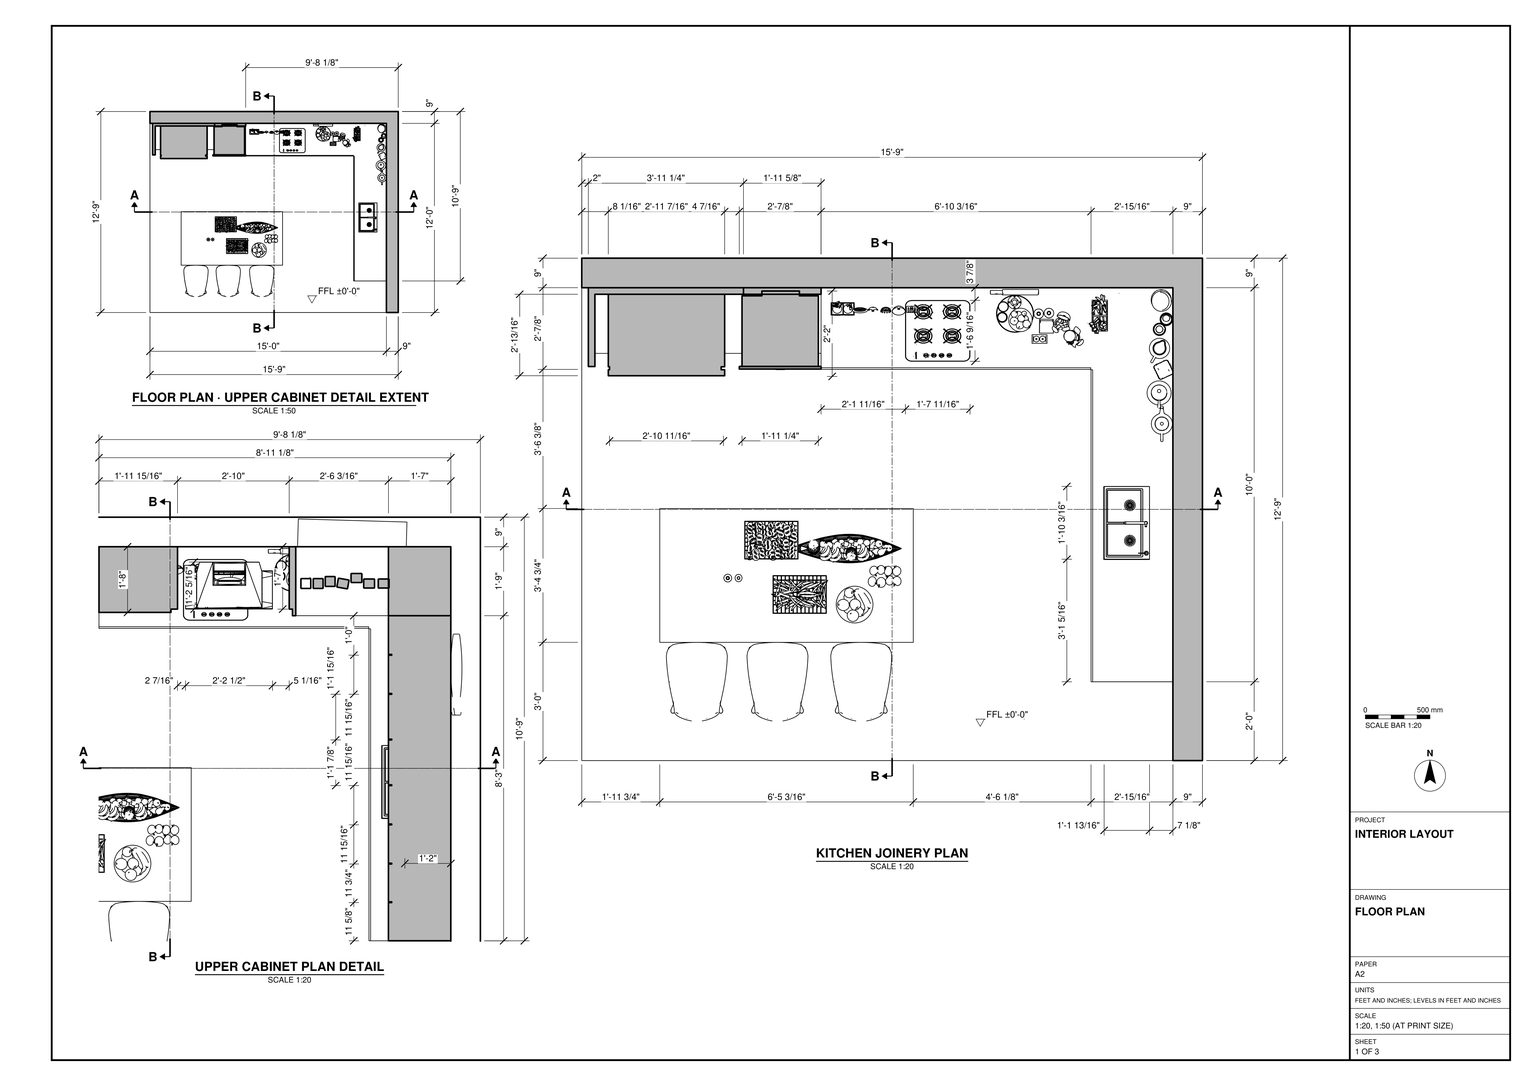
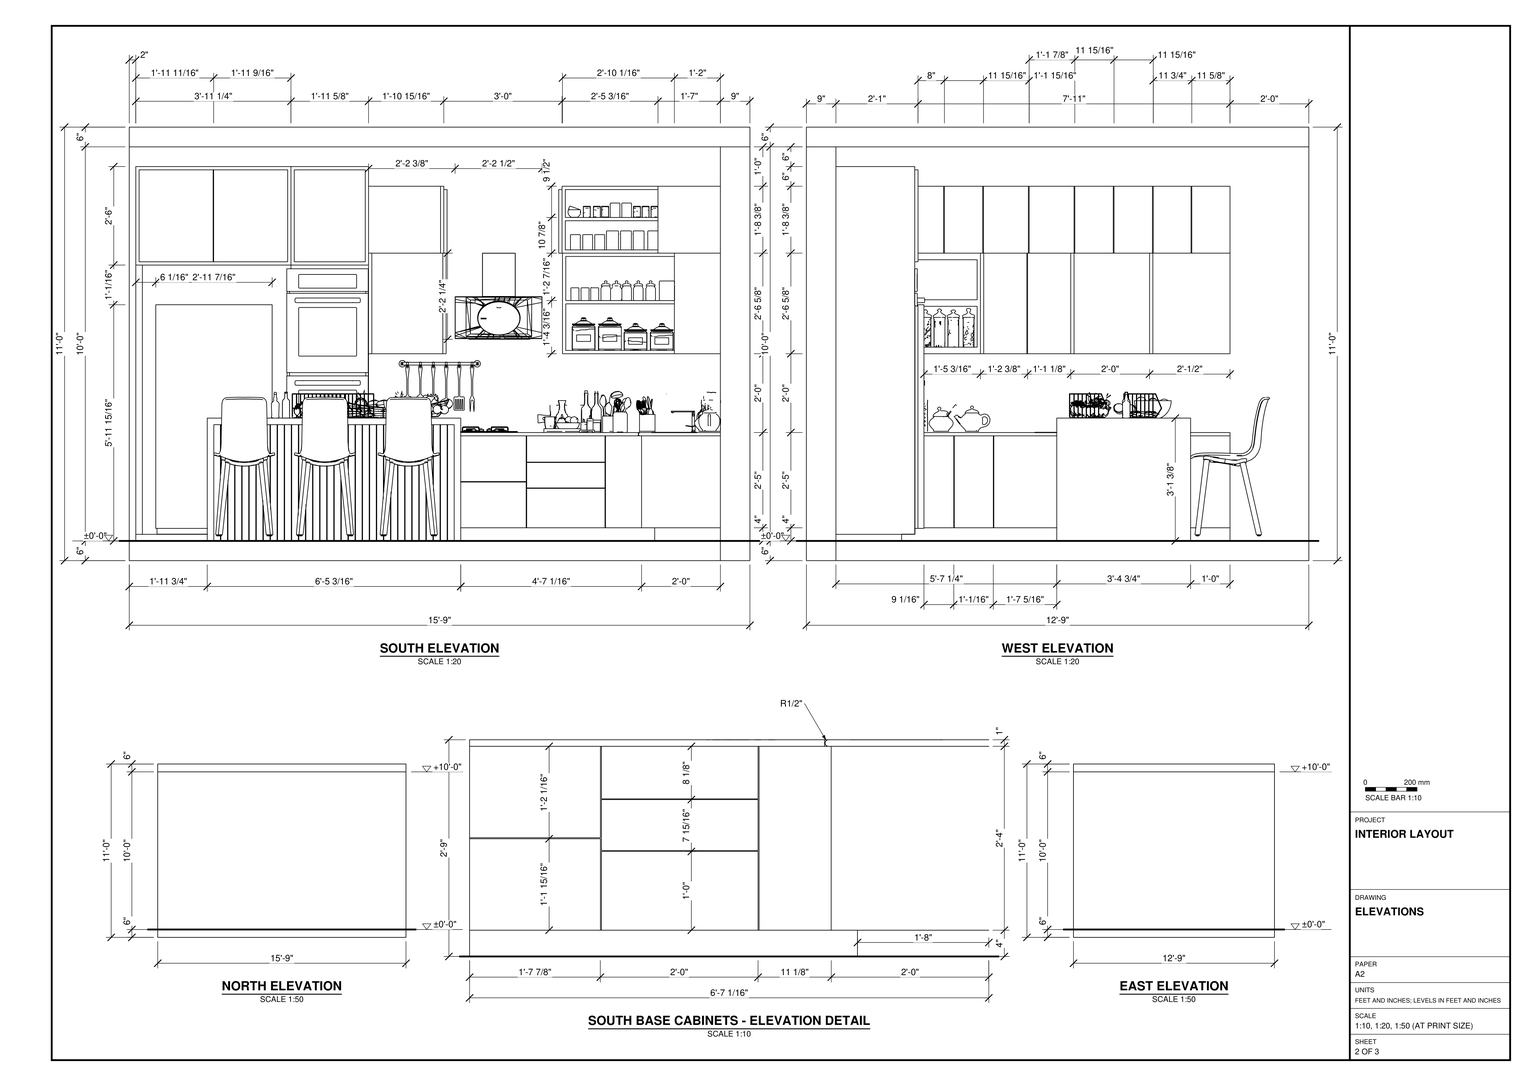
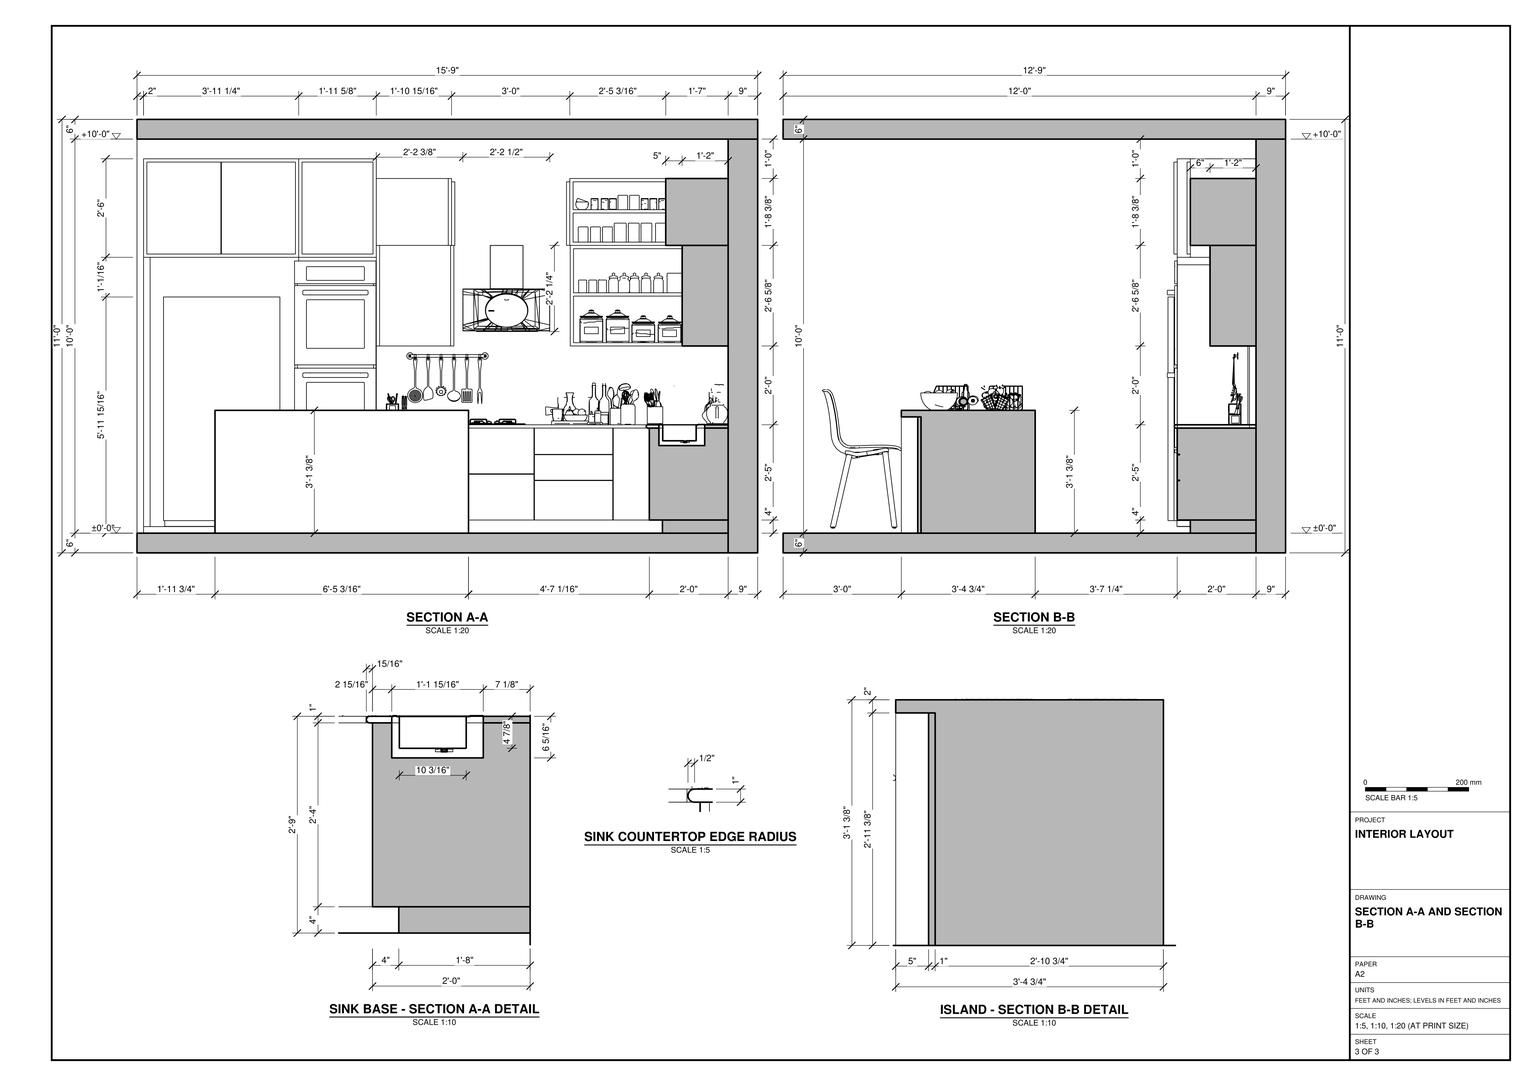
Build the kitchen in SketchUp from task_files/diagram_01.pdf. Work in feet and inches. The overall model is 15'-9" wide, 12'-9" deep and 11'-0" high, with the finished floor at ±0'-0". Model the 9" back and right-hand walls, leaving the other two sides open as drawn. Include the 6" floor and overhead slabs with 10'-0" clear between them.

Use the plan to lay out the tall appliance bays and cooking counter along the back wall, with the sink counter returning along the right-hand wall. Follow the elevations for the cupboard fronts, drawer divisions, open shelves and upper cabinets. Place the cooktop beneath the hood and fit the double-bowl sink into the return. Use the enlarged sections for the recessed base, countertop edge and island overhang.

Set the island parallel to the back wall, with three seats along the long edge facing the cooking area. Decor and loose items, including countertop accessories and appliances, may be any suitable library components placed as shown. Keep the walls, slabs and each furniture or joinery piece in separate groups or components, and use components for repeated parts. Save one SketchUp model as output_files/kitchen_with_l_shaped_cabinetry_and_seating_island.skp.

# SketchUp Ruby script. Lengths in inches.
U = 1.inch
M = Sketchup.active_model
def pt(a) = Geom::Point3d.new(a.map { |v| v * U })
def face(e, loops, mat)
  f = e.add_face(loops[0].map { |a| pt(a) })
  loops[1..].each { |l| e.add_face(l.map { |a| pt(a) }).erase! }
  f.material = f.back_material = mat if mat
  f
end
# faces: each face lists its corners as indices into pts; further lists are holes
def faces(e, pts, list, mat = nil) = list.each { |f| face(e, (f[0].is_a?(Array) ? f : [f]).map { |l| l.map { |i| pts[i] } }, mat) }
# xy, xz, yz: faces in a plane at the given z, y or x. An outline is a flat list of corners, or four numbers for a rectangle; further outlines are holes
def ring(l) = l.size == 4 ? [[l[0], l[1]], [l[2], l[1]], [l[2], l[3]], [l[0], l[3]]] : l.each_slice(2).to_a
def flat(e, list, mat, &to3) = list.each { |f| face(e, (f[0].is_a?(Array) ? f : [f]).map { |l| ring(l).map { |u, v| to3.(u, v) } }, mat) }
def xy(e, z, list, mat = nil) = flat(e, list, mat) { |x, y| [x, y, z] }
def xz(e, y, list, mat = nil) = flat(e, list, mat) { |x, z| [x, y, z] }
def yz(e, x, list, mat = nil) = flat(e, list, mat) { |y, z| [x, y, z] }
def lines(e, pts, list) = list.each { |a, b| e.add_line(pt(pts[a]), pt(pts[b])) }
# prism: a flat outline (further loops are holes) pulled along v
def prism(e, loops, v, mat = nil)
  f = face(e, loops, mat); d = Geom::Vector3d.new(v.map { |x| x * U })
  f.pushpull(f.normal.samedirection?(d) ? d.length : -d.length)
end
def box(e, o, s, mat = nil) = prism(e, [[o, [o[0] + s[0], o[1], o[2]], [o[0] + s[0], o[1] + s[1], o[2]], [o[0], o[1] + s[1], o[2]]]], [0, 0, s[2]], mat)
def at(x, y, z, deg = 0) = Geom::Transformation.translation(pt([x, y, z])) * Geom::Transformation.rotation(ORIGIN, Z_AXIS, deg.degrees)
def axes(o, x, y, z) = Geom::Transformation.new([*x, 0, *y, 0, *z, 0, *pt(o).to_a, 1])
def part(name) = M.definitions.add(name)
# library, detail: a bought-in or finely detailed component or shape, given as its bounding box
def library(name, o, s) = part(name).tap { |d| box(d.entities, o, s) }
def detail(e, o, s) = box(e.add_group.entities, o, s)
def put(e, d, t, mat = nil) = e.add_instance(d, t).tap { |i| i.material = mat if mat }
def group(e, t, mat = nil) = e.add_group.tap { |g| g.transformation = t; g.material = mat if mat }.entities
root = M.entities
M.materials.add("Ceramic_cream_1").color = [121, 112, 98]
M.materials.add("Glass Realtime1").color = [156, 156, 156]
M.materials["Glass Realtime1"].alpha = 0.15
M.materials.add("Metal Black1").color = [54, 53, 53]
M.materials.add("Metal_Seamed1").color = [118, 119, 115]
M.materials.add("[Metal_Aluminum_Anodized]1").color = [202, 209, 219]
M.materials.add("ceramic_Apothecary1").color = [254, 254, 254]
M.materials.add("storage dark green").color = [51, 102, 0]
M.materials.add("utensils_wood_1").color = [176, 135, 87]
M.materials.add("utensils_wood_2").color = [89, 58, 24]
c1 = part("Fiher Paykal 3 D Fridge")
xy(c1.entities,0,[[0,0,0,35.43,22.07,35.43,22.07,34.37,22.97,34.37,22.97,35.43,24.8,35.43,24.8,0,22.97,0,22.97,0.375,22.07,0.375,22.07,0]])
xy(c1.entities,67.74,[[22.07,0.375,22.97,34.37]],"[Metal_Aluminum_Anodized]1")
xy(c1.entities,68.11,[[0,0,22.07,35.43],[22.97,0,24.8,35.43]],"[Metal_Aluminum_Anodized]1")
xz(c1.entities,0,[[0,0,22.07,68.11],[22.97,0,24.8,68.11]],"[Metal_Aluminum_Anodized]1")
xz(c1.entities,0.375,[[22.07,0,22.97,67.74]],"[Metal_Aluminum_Anodized]1")
xz(c1.entities,34.37,[[22.07,0,22.97,67.74]],"[Metal_Aluminum_Anodized]1")
xz(c1.entities,35.43,[[0,0,22.07,68.11],[22.97,0,24.8,68.11]],"[Metal_Aluminum_Anodized]1")
yz(c1.entities,0,[[0,0,35.43,68.11]])
yz(c1.entities,22.07,[[0,0,0.375,67.74],[34.37,0,35.43,68.11],[0,67.74,34.37,68.11]],"[Metal_Aluminum_Anodized]1")
yz(c1.entities,22.97,[[0,0,0.375,67.74],[34.37,0,35.43,68.11],[0,67.74,34.37,68.11]],"[Metal_Aluminum_Anodized]1")
yz(c1.entities,24.8,[[0,0,35.43,68.11]])
c2 = part("Refrigerator shelf")
box(c2.entities,[0,-3.3,-0.8125],[22.07,34.68,1.75])
c3 = part("Fisher Paykal fridge with water")
put(c3.entities,c1,at(0,0,1.75))
put(c3.entities,c2,at(0,3.67,0.8125),"Metal_Seamed1")
c4 = part("Fisher Paylal fridge with water")
put(c4.entities,c3,at(17.54,30.6875,0))
c5 = library("Component",[-0.02,-19.69,0],[22.64,19.69,1.77])
c6 = library("Kitchen washbasin",[0,0,-0.81],[20.87,33.47,18.01])
c7 = library("Chimney",[0,-14.34,0],[33.95,14.34,33.72])
c8 = library("chair01",[0,0,0],[19.41,18.57,31.29])
c9 = library("utensil 8",[0,0,0],[7.12,4.41,9.55])
c10 = library("Glass_Apothecary_Jar",[-11.5,-3.52,0],[30.82,7.02,10])
c11 = library("skpD5F4",[0,-2.85,-0.14],[24.79,2.85,15.53])
c12 = library("KITCHEN UTENSILS",[-13.1875,41.6,-0.19],[9.62,14.28,11.99])
c13 = library("hruska 3",[0,0,0],[2.49,2.49,4.3])
c14 = library("jablko 8",[-1.43,-1.43,0.02],[2.86,2.86,3.5])
c15 = library("jablko zelene 2",[-1.02,-1.3,0.02],[2.55,2.56,3.49])
c16 = library("Fruit bowl",[0,0,0],[64.45,17.87,11.51])
c17 = library("Fruit assortment",[-0.25,2.66,-0.93],[43.16,13.75,13.67])
c18 = part("Fruit bowl centerpiece")
put(c18.entities,c13,axes([191.04,13.07,47.69],[1.63064,1.10312,-5.75014],[-3.40555,5.03411,0],[4.7627,3.22194,1.96871]))
put(c18.entities,c14,axes([209.5,34.72,23.18],[5.70033,0,-2.10862],[0,6.07783,0],[2.10862,0,5.70033]))
put(c18.entities,c15,axes([211.07,36.17,27.83],[4.91404,0.76073,3.49478],[-0.92982,6.00628,0],[-3.45364,-0.53465,4.97257]))
put(c18.entities,c13,axes([189.28,29.03,22.03],[6.07783,0,0],[0,5.77394,0],[0,0,6.07783]))
put(c18.entities,c13,axes([185.58,31.01,18.15],[0.72274,-5.85231,1.47245],[4.01879,1.57306,4.27958],[-4.50188,0.46472,4.05673]))
put(c18.entities,c14,axes([183.64,42.01,28.15],[-2.8871,2.25339,3.57],[0.37031,-4.08542,2.8782],[4.20389,1.92165,2.18678]))
put(c18.entities,c15,axes([184.64,40.56,22.47],[4.63786,0,2.10399],[0,5.39237,0],[-2.10399,0,4.63786]))
put(c18.entities,c14,axes([185.4375,44.76,36.36],[3.25338,-4.91707,-1.4758],[4.47789,3.57246,-2.03126],[2.51078,0,5.53498]))
put(c18.entities,c16,axes([0,0,0],[3.75871,0,0],[0,3.75871,0],[0,0,3.75871]))
put(c18.entities,c17,axes([20.93,-11.64,13.28],[4.34131,0,0],[0,4.34131,0],[0,0,4.34131]))
c19 = library("vm_v2_031",[-7.89,-7.89,0],[15.78,15.78,6.41])
c20 = library("wine (1)",[0,0,0],[5.57,2.41,7.92])
c21 = part("Group\#16")
box(c21.entities,[0,0,0],[2,1,35.4])
c22 = part("Difference\#1")
xy(c22.entities,0,[[156,0,156,23.92,156.71,23.92,156.71,24.08,156,24.08,156,35.92,156.71,35.92,156.71,36.08,156,36.08,156,47.92,156.71,47.92,156.71,48.08,156,48.08,156,71.92,156.71,71.92,156.71,72.08,156,72.08,156,83.96,156.71,83.96,156.71,84.12,156,84.12,156,96,145.02,96,145.02,96.71,144.87,96.71,144.87,96,121.02,96,121.02,96.71,120.87,96.71,120.87,96,97.02,96,97.02,96.71,96.75,96.71,96.75,96,72.98,96,72.98,96.71,72.87,96.71,72.87,120,180,120,180,0]])
xy(c22.entities,12,[[72.98,96,96.75,96.71],[121.02,96,144.87,96.71]])
xy(c22.entities,12.12,[[72.98,96,96.75,96.71]])
xy(c22.entities,12.13,[[121.02,96,144.87,96.71]])
xy(c22.entities,13.92,[[97.02,96,120.87,96.71]])
xy(c22.entities,14.08,[[97.02,96,120.87,96.71]])
xy(c22.entities,19.88,[[72.98,96,96.75,96.71],[121.02,96,144.87,96.71]])
xy(c22.entities,20,[[72.98,96,96.75,96.71],[121.02,96,144.87,96.71]])
xy(c22.entities,22.67,[[158.93,37.21,172.87,59.45]])
xy(c22.entities,28,[[[156,0,180,0,180,120,72.87,120,72.87,96.71,72.98,96.71,72.98,96,96.75,96,96.75,96.71,97.02,96.71,97.02,96,120.87,96,120.87,96.71,121.02,96.71,121.02,96,144.87,96,144.87,96.71,145.02,96.71,145.02,96,156,96,156,84.12,156.71,84.12,156.71,83.96,156,83.96,156,72.08,156.71,72.08,156.71,71.92,156,71.92,156,48.08,156.71,48.08,156.71,47.92,156,47.92,156,36.08,156.71,36.08,156.71,35.92,156,35.92,156,24.08,156.71,24.08,156.71,23.92,156,23.92],[158.93,37.21,172.87,59.45]]])
xz(c22.entities,0,[[156,0,180,28]])
xz(c22.entities,23.92,[[156,0,156.71,28]])
xz(c22.entities,24.08,[[156,0,156.71,28]])
xz(c22.entities,35.92,[[156,0,156.71,28]])
xz(c22.entities,36.08,[[156,0,156.71,28]])
xz(c22.entities,37.21,[[158.93,22.67,172.87,28]])
xz(c22.entities,47.92,[[156,0,156.71,28]])
xz(c22.entities,48.08,[[156,0,156.71,28]])
xz(c22.entities,59.45,[[158.93,22.67,172.87,28]])
xz(c22.entities,71.92,[[156,0,156.71,28]])
xz(c22.entities,72.08,[[156,0,156.71,28]])
xz(c22.entities,83.96,[[156,0,156.71,28]])
xz(c22.entities,84.12,[[156,0,156.71,28]])
xz(c22.entities,96,[[72.98,0,96.75,12],[97.02,0,120.87,13.92],[121.02,0,144.87,12],[145.02,0,156,28],[72.98,12.12,96.75,19.88],
  [121.02,12.13,144.87,19.88],[97.02,14.08,120.87,28],[72.98,20,96.75,28],[121.02,20,144.87,28]])
xz(c22.entities,96.71,[[[72.87,0,72.98,0,72.98,12,96.75,12,96.75,0,97.02,0,97.02,13.92,120.87,13.92,120.87,0,121.02,0,121.02,12,144.87,12,144.87,0,145.02,0,145.02,28,144.87,28,144.87,20,121.02,20,121.02,28,120.87,28,120.87,14.08,97.02,14.08,97.02,28,96.75,28,96.75,20,72.98,20,72.98,28,72.87,28],[121.02,12.13,144.87,19.88],[72.98,12.12,96.75,19.88]]])
xz(c22.entities,120,[[72.87,0,180,28]])
yz(c22.entities,72.87,[[96.71,0,120,28]])
yz(c22.entities,72.98,[[96,0,96.71,12],[96,12.12,96.71,19.88],[96,20,96.71,28]])
yz(c22.entities,96.75,[[96,0,96.71,12],[96,12.12,96.71,19.88],[96,20,96.71,28]])
yz(c22.entities,97.02,[[96,0,96.71,13.92],[96,14.08,96.71,28]])
yz(c22.entities,120.87,[[96,0,96.71,13.92],[96,14.08,96.71,28]])
yz(c22.entities,121.02,[[96,0,96.71,12],[96,12.13,96.71,19.88],[96,20,96.71,28]])
yz(c22.entities,144.87,[[96,0,96.71,12],[96,12.13,96.71,19.88],[96,20,96.71,28]])
yz(c22.entities,145.02,[[96,0,96.71,28]])
yz(c22.entities,156,[[0,0,23.92,28],[24.08,0,35.92,28],[36.08,0,47.92,28],[48.08,0,71.92,28],[72.08,0,83.96,28],
  [84.12,0,96,28]])
yz(c22.entities,156.71,[[23.92,0,24.08,28],[35.92,0,36.08,28],[47.92,0,48.08,28],[71.92,0,72.08,28],[83.96,0,84.12,28]])
yz(c22.entities,158.93,[[37.21,22.67,59.45,28]])
yz(c22.entities,172.87,[[37.21,22.67,59.45,28]])
yz(c22.entities,180,[[0,0,120,28]])
c23 = library("Group\#4",[0,0,0],[30,26,50.75])
c24 = part("Difference")
xy(c24.entities,0,[[[155.57,0,155.57,95,155,95,155,95.63,72.87,95.63,72.87,120,180,120,180,0],[158.93,37.21,172.87,59.45]],[155.52,0,155.57,95],[72.87,95.5625,155,95.6],[72.87,95.6,155,95.63]])
xy(c24.entities,1,[[[155.57,0,180,0,180,120,72.87,120,72.87,95.63,155,95.63,155,95,155.57,95],[158.93,37.21,172.87,59.45]],[155.52,0,155.57,95],[72.87,95.5625,155,95.6],[72.87,95.6,155,95.63]])
xz(c24.entities,0,[[155.52,0,180,0,180,1,155.52,1,155.42,0.98,155.37,0.96,155.32,0.93,155.24,0.87,155.2,0.83,155.14,0.75,155.1,0.65,155.07,0.5,155.1,0.35,155.14,0.25,155.2,0.17,155.24,0.13,155.32,0.07,155.37,0.04,155.42,0.02]])
xz(c24.entities,37.21,[[158.93,0,172.87,1]])
xz(c24.entities,59.45,[[158.93,0,172.87,1]])
xz(c24.entities,95,[[155,0,155.57,0,155.52,0,155.42,0.02,155.37,0.04,155.32,0.07,155.24,0.13,155.2,0.17,155.14,0.25,155.1,0.35,155.07,0.5,155.1,0.65,155.14,0.75,155.2,0.83,155.24,0.87,155.32,0.93,155.37,0.96,155.42,0.98,155.52,1,155.57,1,155,1]])
xz(c24.entities,95.13,[[72.87,0.45,155,0.48],[72.87,0.48,155,0.52],[72.87,0.52,155,0.55]])
xz(c24.entities,120,[[72.87,0,180,1]])
yz(c24.entities,72.87,[[95.5625,0,95.53,0.01,95.49,0.02,95.43,0.04,95.34,0.1,95.3125,0.12,95.28,0.14,95.26,0.17,95.24,0.19,95.18,0.28,95.17,0.3125,95.16,0.35,95.14,0.41,95.13,0.45,95.13,0.55,95.14,0.59,95.16,0.65,95.17,0.6875,95.18,0.72,95.24,0.81,95.26,0.83,95.28,0.86,95.3125,0.88,95.34,0.9,95.43,0.96,95.49,0.98,95.53,0.99,95.5625,1,120,1,120,0]])
yz(c24.entities,155,[[95,0,95,1,95.63,1,95.5625,1,95.53,0.99,95.49,0.98,95.43,0.96,95.34,0.9,95.3125,0.88,95.28,0.86,95.26,0.83,95.24,0.81,95.18,0.72,95.17,0.6875,95.16,0.65,95.14,0.59,95.13,0.55,95.13,0.45,95.14,0.41,95.16,0.35,95.17,0.3125,95.18,0.28,95.24,0.19,95.26,0.17,95.28,0.14,95.3125,0.12,95.34,0.1,95.43,0.04,95.49,0.02,95.53,0.01,95.5625,0,95.63,0]])
yz(c24.entities,158.93,[[37.21,0,59.45,1]])
yz(c24.entities,172.87,[[37.21,0,59.45,1]])
yz(c24.entities,180,[[0,0,120,1]])
p = [[155.37,0,0.04],[155.32,0,0.07],[155.32,95,0.07],[155.37,95,0.04],[155.42,0,0.02],[155.42,95,0.02],
  [155.47,0,0.01],[155.47,95,0.01],[155.52,0,0],[155.52,95,0],[72.87,95.43,0.04],[72.87,95.46,0.03],
  [155,95.46,0.03],[155,95.43,0.04],[72.87,95.4,0.06],[155,95.4,0.06],[72.87,95.53,0.01],[72.87,95.5625,0],
  [155,95.5625,0],[155,95.53,0.01],[72.87,95.49,0.02],[155,95.49,0.02],[155.24,0,0.13],[155.2,0,0.17],
  [155.2,95,0.17],[155.24,95,0.13],[155.28,0,0.1],[155.28,95,0.1],[72.87,95.34,0.1],[72.87,95.37,0.08],
  [155,95.37,0.08],[155,95.34,0.1],[72.87,95.3125,0.12],[155,95.3125,0.12],[72.87,95.28,0.14],[155,95.28,0.14],
  [72.87,95.26,0.17],[155,95.26,0.17],[155.14,0,0.25],[155.12,0,0.3],[155.12,95,0.3],[155.14,95,0.25],
  [155.17,0,0.21],[155.17,95,0.21],[72.87,95.24,0.19],[155,95.24,0.19],[72.87,95.22,0.22],[155,95.22,0.22],
  [72.87,95.2,0.25],[155,95.2,0.25],[72.87,95.18,0.28],[155,95.18,0.28],[155.1,0,0.35],[155.09,0,0.4],
  [155.09,95,0.4],[155.1,95,0.35],[72.87,95.15,0.38],[72.87,95.16,0.35],[155,95.16,0.35],[155,95.15,0.38],
  [72.87,95.17,0.3125],[155,95.17,0.3125],[155.08,0,0.45],[155.07,0,0.5],[155.07,95,0.5],[155.08,95,0.45],
  [72.87,95.14,0.41],[155,95.14,0.41],[72.87,95.13,0.45],[155,95.13,0.45],[155.08,0,0.55],[155.08,95,0.55],
  [155.09,0,0.6],[155.1,0,0.65],[155.1,95,0.65],[155.09,95,0.6],[72.87,95.14,0.59],[72.87,95.13,0.55],
  [155,95.13,0.55],[155,95.14,0.59],[72.87,95.15,0.62],[155,95.15,0.62],[72.87,95.16,0.65],[155,95.16,0.65],
  [155.12,0,0.7],[155.14,0,0.75],[155.14,95,0.75],[155.12,95,0.7],[72.87,95.17,0.6875],[155,95.17,0.6875],
  [72.87,95.18,0.72],[155,95.18,0.72],[72.87,95.2,0.75],[155,95.2,0.75],[155.17,0,0.79],[155.17,95,0.79],
  [155.2,0,0.83],[155.24,0,0.87],[155.24,95,0.87],[155.2,95,0.83],[72.87,95.22,0.78],[155,95.22,0.78],
  [72.87,95.24,0.81],[155,95.24,0.81],[72.87,95.26,0.83],[155,95.26,0.83],[72.87,95.28,0.86],[155,95.28,0.86],
  [155.28,0,0.9],[155.28,95,0.9],[155.32,0,0.93],[155.37,0,0.96],[155.37,95,0.96],[155.32,95,0.93],
  [72.87,95.3125,0.88],[155,95.3125,0.88],[72.87,95.34,0.9],[155,95.34,0.9],[72.87,95.37,0.92],[155,95.37,0.92],
  [72.87,95.4,0.94],[155,95.4,0.94],[72.87,95.43,0.96],[155,95.43,0.96],[155.42,0,0.98],[155.47,0,0.99],
  [155.47,95,0.99],[155.42,95,0.98],[155.52,0,1],[155.52,95,1],[72.87,95.46,0.97],[155,95.46,0.97],
  [72.87,95.49,0.98],[155,95.49,0.98],[72.87,95.53,0.99],[155,95.53,0.99],[72.87,95.5625,1],[155,95.5625,1]]
faces(c24.entities,p,[[0,1,2,3],[4,0,3,5],[6,4,5,7],[8,6,7,9],[10,11,12,13],[14,10,13,15],[16,17,18,19],[20,16,19,21],
  [11,20,21,12],[22,23,24,25],[26,22,25,27],[1,26,27,2],[28,29,30,31],[32,28,31,33],[34,32,33,35],[36,34,35,37],
  [29,14,15,30],[38,39,40,41],[42,38,41,43],[23,42,43,24],[44,36,37,45],[46,44,45,47],[48,46,47,49],[50,48,49,51],
  [52,53,54,55],[39,52,55,40],[56,57,58,59],[60,50,51,61],[57,60,61,58],[62,63,64,65],[53,62,65,54],[66,56,59,67],
  [68,66,67,69],[63,70,71,64],[72,73,74,75],[70,72,75,71],[76,77,78,79],[80,76,79,81],[82,80,81,83],[84,85,86,87],
  [73,84,87,74],[88,82,83,89],[90,88,89,91],[92,90,91,93],[85,94,95,86],[96,97,98,99],[94,96,99,95],[100,92,93,101],
  [102,100,101,103],[104,102,103,105],[106,104,105,107],[97,108,109,98],[110,111,112,113],[108,110,113,109],[114,106,107,115],[116,114,115,117],
  [118,116,117,119],[120,118,119,121],[122,120,121,123],[124,125,126,127],[111,124,127,112],[125,128,129,126],[130,122,123,131],[132,130,131,133],
  [134,132,133,135],[136,134,135,137]])
c25 = library("Group\#77",[-332.7,68.71,378.69],[103.45,103.45,159.72])
c26 = library("Group\#78",[-457.8,68.7,378.69],[103.44,103.46,159.72])
c27 = library("Group\#79",[-210.76,89.58,378.69],[103.46,103.45,159.72])
c28 = library("Group\#80",[-462.66,84.21,613.65],[72.44,72.44,111.8])
c29 = library("Group\#81",[-374.05,84.21,613.65],[72.44,72.44,111.8])
c30 = library("Group\#82",[-289.4,84.22,613.65],[72.44,72.43,111.8])
c31 = library("Group\#83",[-92.73,64.66,378.72],[126.77,111.9,197.69])
c32 = library("Group\#84",[51.24,128.79,378.72],[113.79,95.47,197.69])
c33 = library("Group\#85",[179.9,72.7,378.72],[113.8,95.46,197.69])
c34 = library("Group\#86",[327.72,72.7,378.72],[113.79,95.46,197.69])
c35 = library("Group\#88",[309.63,77.04,613.73],[136.79,86.78,171.39])
c36 = library("Group\#89",[-198.8,84.74,613.85],[84,84,172.39])
c37 = library("Group\#90",[-105.26,84.74,613.85],[84,84,172.39])
c38 = library("Group\#91",[-15.73,84.74,613.85],[84,84,172.39])
c39 = library("Group\#92",[85.42,84.74,613.85],[84,84,172.42])
c40 = library("Group\#93",[193.57,84.74,613.85],[84,84,172.39])
c41 = library("Group\#94",[-504.125,120.57,-0.1],[108.2,108.21,338.13])
c42 = library("Group\#95",[-376.9,120.94,-0.1],[107.79,107.8,326.37])
c43 = library("Group\#96",[-254.81,120.48,-0.6],[108.21,108.21,334.5])
c44 = library("Group\#97",[-133.01,121.19,-0.1],[106.95,106.95,324.89])
c45 = library("Group\#98",[0.46,121.12,-0.1],[106.94,106.94,338.14])
c46 = library("Group\#136",[-410.5,-181.74,316.41],[112.68,105.63,132.85])
c47 = library("Group\#135",[-77.16,-243.45,0.06],[77.78,77.39,334.5])
c48 = library("Group\#134",[5.16,-238.13,0.06],[77.38,77.77,330.87])
c49 = library("Group\#133",[-32.31,-359.75,0.0625],[113.14,110.83,100])
c50 = library("Group\#132",[-378.93,-184.58,554.39],[111.07,111.08,100.74])
c51 = library("Group\#131",[-8.64,-128.96,554.5],[87.78,87.84,126.93])
c52 = library("Group\#130",[63.24,-202.95,316.58],[142.19,125.22,138.6])
c53 = library("Group\#129",[-158.11,-190.97,316.58],[127.96,105.64,110.41])
c54 = library("Group\#128",[33.26,-68.65,316.32],[420.74,57.7,172.99])
c55 = library("Group\#127",[-424.81,-54.29,0.29],[386.66,43.55,222.03])
c56 = library("Group\#126",[93.54,-167.13,554.5],[87.79,87.86,126.93])
c57 = library("Group\#125",[-44.89,-168.51,316.32],[101.05,102.35,203.58])
c58 = library("Group\#124",[-290.0625,-171.35,316.41],[118.25,100.67,149.82])
c59 = library("Group\#123",[193.54,-180.875,316.58],[185.99,109.56,131.55])
c60 = library("Group\#122",[-375.96,-353.73,0.05],[297.45,297.44,31.27])
c61 = library("Group\#121",[-278.11,-348.23,5.8],[187.87,187.87,121.65])
c62 = library("Group\#120",[-284.5,-166.25,5.875],[106.63,106.63,250.48])
c63 = library("Group\#119",[-370.5625,-274.21,5.8125],[90.77,166.34,120.375])
c64 = library("Group\#118",[70.49,-356.56,0.0625],[143.03,166.7,314.72])
c65 = library("Group\#117",[162.6875,-473.8,0.53],[157.34,166.37,329.78])
c66 = library("Group\#116",[-91.3125,-441.93,-0.01],[120,70.11,138.07])
c67 = library("Group\#115",[-244.67,-166.72,554.3125],[62.14,62.13,98.96])
c68 = library("Group\#114",[-155.46,-166.74,554.3125],[62.14,62.13,98.96])
c69 = library("Group\#113",[197.13,-153.24,554.3125],[62.13,62.13,98.96])
c70 = library("Group\#101",[-83.17,-142.88,554.3125],[62.13,62.13,98.96])
c71 = library("Group\#100",[351.36,-159.89,554.3125],[62.1,62.11,98.96])
c72 = library("Group\#99",[273.08,-166.73,554.3125],[62.1,62.12,98.96])
c73 = library("Group\#240",[-0.73,-0.29,-1.22],[12.46,17.33,7.15])
c74 = part("pod 28k")
p = [[-1.32,0.16,0.14],[-1.25,0.58,0],[-0.03,0,0.14],[-0.03,0.53,0],[1.18,0.58,0],[1.25,0.16,0.14],
  [-2.55,0.75,0.0625],[2.375,0.74,0],[2.51,0.33,0.14],[3.59,0.9,0.31],[-1.2,0.84,0.36],[-0.03,0.79,0.36],
  [1.14,0.84,0.36],[-2.48,0.96,0.36],[2.29,0.99,0.36],[-0.03,0,0.58],[-1.32,0.16,0.58],[1.25,0.16,0.58],
  [-2.67,0.41,0.17],[-2.67,0.41,0.54],[2.51,0.33,0.58],[-3.54,0.92,0.27],[-3.5,0.98,0.36],[-3.59,0.82,0.41],
  [-3.59,0.82,0.3],[2.375,0.74,0.72],[-3.54,0.92,0.45],[-2.55,0.75,0.66],[-1.25,0.58,0.72],[-0.03,0.53,0.72],
  [1.18,0.58,0.72]]
faces(c74.entities,p,[[0,1,2],[3,2,1],[3,4,2],[5,2,4],[1,0,6],[4,7,8,5],[9,8,7],[1,10,11,3],
  [3,11,12,4],[6,13,1],[10,1,13],[4,12,14,7],[9,7,14],[2,15,16,0],[5,17,15,2],[18,6,0],
  [0,16,19,18],[8,20,17,5],[8,9,20],[6,18,21],[13,6,22],[21,22,6],[18,19,23,24],[24,21,18],
  [9,25,20],[9,14,25],[23,26,22,21,24],[23,19,26],[27,26,19],[10,28,29,11],[11,29,30,12],[28,10,27],
  [12,30,25,14],[26,27,22],[13,22,27],[13,27,10],[19,16,27],[16,15,28],[29,28,15],[15,17,29],
  [28,27,16],[30,29,17],[17,20,25,30]],"storage dark green")
c75 = part("Group131\#5")
put(c75.entities,c74,axes([0.88,13.28,1.97],[0.08806,-1.13493,0],[-1.12727,-0.08747,0.13203],[-0.13163,-0.01021,-1.13066]))
put(c75.entities,c74,axes([-3.27,11.34,2.22],[-0.41224,0.86298,-0.03879],[0.86341,0.41299,0.01216],[0.0277,-0.02975,-0.95631]))
put(c75.entities,c74,axes([-0.99,17.3,1.22],[-0.96177,-0.07847,-0.06756],[-0.08625,0.95635,0.11701],[0.0573,0.12236,-0.95785]))
put(c75.entities,c74,axes([-2.69,17.01,1.36],[-0.74478,0.41699,-0.05118],[0.4137,0.74607,0.0585],[0.07318,0.02619,-0.85156]))
put(c75.entities,c74,axes([-2.61,4.95,1.14],[-0.25029,-0.96482,-0.11129],[-0.96955,0.25496,-0.02982],[0.05698,0.10014,-0.99631]))
put(c75.entities,c74,axes([-1.62,5.4,1.7],[-0.76917,0.09582,0.04319],[0.09175,0.76774,-0.06943],[-0.05128,-0.06369,-0.772]))
put(c75.entities,c74,axes([-0.04,1.51,1.46],[-1.09474,-0.1947,-0.16224],[-0.21897,1.08881,0.17094],[0.12759,0.19815,-1.0987]))
put(c75.entities,c74,axes([1.91,17.06,1.74],[0.73958,-0.26099,0.05468],[-0.26497,-0.7374,0.06414],[0.02999,-0.07877,-0.78165]))
put(c75.entities,c74,axes([-1.83,12.62,1.61],[0.43066,-0.82776,0],[-0.82738,-0.43046,-0.0283],[0.0251,0.01306,-0.93266]))
put(c75.entities,c74,axes([1.94,8.19,1.31],[-0.48391,1.1503,-0.06308],[1.14527,0.47295,-0.16126],[-0.12458,-0.12027,-1.23748]))
put(c75.entities,c74,axes([-0.52,3.01,1.19],[0.32522,-0.74877,-0.0965],[-0.75384,-0.32781,0.00304],[-0.04125,0.08729,-0.81635]))
put(c75.entities,c74,axes([1.9375,13.98,1.85],[0.33905,1.11558,0.13471],[1.11919,-0.34783,0.06363],[0.10039,0.11007,-1.16422]))
put(c75.entities,c74,axes([2.64,8.02,1.93],[-0.58533,0.62108,0.10825],[0.62771,0.58788,0.02119],[-0.05868,0.0934,-0.85317]))
put(c75.entities,c74,axes([1.04,5.23,2.02],[-0.28676,-1.1336,0.049],[-1.13465,0.28625,-0.01796],[0.00541,-0.05191,-1.16917]))
put(c75.entities,c74,axes([3.38,9.7,1.25],[-0.48903,-1.12137,-0.08142],[-1.1239,0.48513,0.06885],[-0.03075,0.1021,-1.22142]))
put(c75.entities,c74,axes([2.36,11.16,1.5],[-0.52318,0.57642,-0.01069],[0.57647,0.52323,0.00012],[0.00728,-0.00784,-0.77845]))
put(c75.entities,c74,axes([2.27,4.46,1.73],[0.34833,-0.94898,0.0526],[-0.94945,-0.34999,-0.0268],[0.04331,-0.04012,-1.01053]))
put(c75.entities,c74,axes([3.18,3.01,1.52],[-0.40076,0.67102,-0.00499],[0.67063,0.40071,0.02429],[0.02341,0.00818,-0.78121]))
put(c75.entities,c74,axes([-3.14,8.05,1.93],[-0.58728,0.62805,-0.02701],[0.62771,0.58788,0.02119],[0.03393,-0.00525,-0.85959]))
put(c75.entities,c74,axes([-2.51,14.75,1.74],[-0.58533,0.62108,0.10825],[0.62771,0.58788,0.02119],[-0.05868,0.0934,-0.85317]))
c76 = library("Group147\#4",[-6.07,0,0.26],[12.14,17.53,5.27])
c77 = library("Group\#164",[0,0,0],[11.58,16.3,7.44])
p = [[4,120,84],[2,120,84],[184.03,119.35,14.82],[184.03,119.29,14.82],[184.08,119.29,14.82]]
lines(root,p,[[0,1],[2,3],[3,4],[4,2]])
put(root,c4,at(-22.61,159.54,2.0625,-90))
put(root,c5,axes([118.23,140.13,33],[0,-0.82,0],[1,0,0],[0,0,1]))
put(root,c6,axes([172.89,83.5,28.125],[-0.663,0,0],[0,-0.663,0],[0,0,0.663]))
put(root,c7,axes([99.22,139.34,60.65],[0.78,0,0],[0,1,0],[0,0,0.8]))
put(root,c8,axes([25.75,36,1.5],[0,-1.24,0],[1,0,0],[0,0,1.35]))
put(root,c8,axes([50.3125,36,1.5],[0,-1.24,0],[1,0,0],[0,0,1.35]))
put(root,c8,axes([75.8125,36,1.5],[0,-1.24,0],[1,0,0],[0,0,1.35]))
put(root,c9,at(75.89,135.59,33))
put(root,c10,at(146.35,138.62,58))
put(root,c11,at(82.15,138.51,39.58))
put(root,c12,at(167.15,87.87,33))
put(root,c18,axes([65.77,60.2,37.4],[0.1302,0,0],[0,0.1302,0],[0,0,0.1302]))
put(root,c19,at(83.07,47.51,37.4))
put(root,c20,at(43.25,54.37,37.4))
g1 = group(root,at(0,0,-6))
box(g1,[0,0,0],[180,144,6])
g2 = group(root,at(0,24,0))
prism(g2,[[[160,100,0],[49.24,100,0],[49.24,120,0],[180,120,0],[180,0,0],[160,0,0]]],[0,0,4])
g3 = group(root,at(49.24,124,4))
xy(g3,0,[[0,0,23.62,20]])
xy(g3,14.01,[[0,18,23.62,20]])
xy(g3,20.01,[[0,0,23.62,18]])
xy(g3,80,[[0,0,23.62,18],[0,18,23.62,20]])
xy(g3,81,[[1,-1,22.62,0]])
xy(g3,109,[[1,-1,22.62,0]])
xy(g3,110,[[0,0,23.62,20]])
xz(g3,-1,[[1,81,22.62,109]])
xz(g3,0,[[0,0,23.62,20.01],[[0,80,23.62,110],[1,81,22.62,109]]])
xz(g3,18,[[0,14.01,23.62,20.01],[0,20.01,23.62,80]])
xz(g3,20,[[0,0,23.62,14.01],[0,14.01,23.62,80],[0,80,23.62,110]])
yz(g3,0,[[0,0,0,20.01,18,20.01,18,14.01,20,14.01,20,0],[18,14.01,20,80],[0,80,20,110]])
yz(g3,1,[[-1,81,0,109]])
yz(g3,22.62,[[-1,81,0,109]])
yz(g3,23.62,[[0,0,20,0,20,14.01,18,14.01,18,20.01,0,20.01],[18,14.01,20,80],[0,80,20,110]])
g4 = group(root,at(0,0,-6))
prism(g4,[[[180,144,0],[0,144,0],[0,153,0],[189,153,0],[189,0,0],[180,0,0]]],[0,0,126])
g5 = group(root,at(2,120,0))
box(g5,[0,4,0],[47.24,20,2])
g6 = group(root,at(2,120,2))
xy(g6,0,[[0,0,0,24,47.24,24,47.24,22,2,22,2,0]])
xy(g6,82,[[2,0,47.24,22]])
xy(g6,83,[[1,-1,2,0],[2,-1,23.54,0],[23.7,-1,46.24,0]])
xy(g6,111,[[1,-1,23.54,0],[23.7,-1,46.24,0]])
xy(g6,112,[[0,0,47.24,24]])
xz(g6,-1,[[1,83,23.54,111],[23.7,83,46.24,111]])
xz(g6,0,[[0,0,2,82],[[0,82,47.24,112],[1,83,46.24,111]],[23.54,83,23.7,111]])
xz(g6,22,[[2,0,47.24,82]])
xz(g6,24,[[0,0,47.24,112]])
yz(g6,0,[[0,0,24,112]])
yz(g6,1,[[-1,83,0,111]])
yz(g6,2,[[0,0,22,82]])
yz(g6,23.54,[[-1,83,0,111]])
yz(g6,23.7,[[-1,83,0,111]])
yz(g6,46.24,[[-1,83,0,111]])
yz(g6,47.24,[[22,0,24,0,24,112,0,112,0,82,22,82]])
g7 = group(root,at(72.87,129,57))
prism(g7,[[[0,15,0],[23.62,15,0],[23.62,2,0],[22.62,2,0],[22.62,1,0],[1,1,0],[1,2,0],[0,2,0]]],[0,0,30.625])
xy(g7,1,[[93.13,0.03,93.73,20.96,60.65,21.9,60.05,0.97]])
xy(g7,15.1875,[[93.13,0.03,60.05,0.97,60.65,21.9,93.73,20.96]])
xy(g7,16.1875,[[93.13,0.03,93.78,22.52,60.7,23.46,60.05,0.97]])
xy(g7,29.625,[[93.13,0.03,60.05,0.97,60.7,23.46,93.78,22.52]])
yz(g7,59.06,[[1,0,15,30.625]])
p = [[59.06,1,0],[94.13,0,0],[94.13,0,30.625],[59.06,1,30.625],[60.05,0.97,15.1875],[93.13,0.03,15.1875],
  [93.13,0.03,1],[60.05,0.97,1],[93.13,0.03,29.625],[93.13,0.03,16.1875],[60.05,0.97,16.1875],[60.05,0.97,29.625],
  [93.73,20.96,15.1875],[93.73,20.96,1],[60.65,21.9,1],[60.65,21.9,15.1875],[93.78,22.52,29.625],[93.78,22.52,16.1875],
  [60.7,23.46,16.1875],[60.7,23.46,29.625]]
faces(g7,p,[[[0,1,2,3],[4,5,6,7],[8,9,10,11]],[6,5,12,13],[4,7,14,15],[13,12,15,14],[9,8,16,17],[11,10,18,19],[19,18,17,16]])
g8 = group(root,at(72.87,129,87.625))
xy(g8,0,[[58.92,-6,58.92,-4,57.92,-4,57.92,15,107.13,15,107.13,-6],[0,-5,0,15,23.92,15,23.92,-4,21.92,-4,21.92,-5]])
xy(g8,1,[[59.92,-6,88.13,15]])
xy(g8,9.875,[[59.92,-6,88.13,15]])
xy(g8,10.875,[[59.92,-6,88.13,15]])
xy(g8,19.375,[[59.92,-6,88.13,15],[22.92,-4,23.92,15],[57.92,-4,58.92,15]])
xy(g8,20.375,[[58.92,-6,107.13,15],[0,-5,21.92,-5,21.92,-4,22.92,-4,22.92,15,0,15]])
xz(g8,-6,[[[58.92,0,89.13,20.375],[59.92,1,88.13,9.875],[59.92,10.875,88.13,19.375]],[89.13,0,107.13,20.375]])
xz(g8,-5,[[0,0,21.92,20.375]])
xz(g8,-4,[[21.92,0,22.92,20.375],[22.92,0,23.92,19.375],[57.92,0,58.92,19.375]])
xz(g8,15,[[0,0,0,20.375,22.92,20.375,22.92,19.375,23.92,19.375,23.92,0],[[57.92,0,57.92,19.375,58.92,19.375,58.92,20.375,107.13,20.375,107.13,0],[59.92,1,88.13,9.875],[59.92,10.875,88.13,19.375]]])
yz(g8,0,[[-5,0,15,20.375]])
yz(g8,21.92,[[-5,0,-4,20.375]])
yz(g8,22.92,[[-4,19.375,15,20.375]])
yz(g8,23.92,[[-4,0,15,19.375]])
yz(g8,57.92,[[-4,0,15,19.375]])
yz(g8,58.92,[[-6,0,-4,20.375],[-4,19.375,15,20.375]])
yz(g8,59.92,[[-6,1,15,9.875],[-6,10.875,15,19.375]])
yz(g8,88.13,[[-6,1,15,9.875],[-6,10.875,15,19.375]])
yz(g8,107.13,[[-6,0,15,20.375]])
g9 = group(root,at(167,24,57))
xy(g9,0,[[-1,0,-1,23.5,0,23.5,0,24.5,-1,24.5,-1,47.5,0,47.5,0,48.5,-1,48.5,-1,61.63,0,61.63,0,61.87,-1,61.87,-1,75,0,75,0,76,-1,76,-1,105,13,105,13,0]])
xy(g9,2,[[-1,77,13,103]])
xy(g9,14.4375,[[-1,77,13,103]])
xy(g9,16.4375,[[-1,77,13,103]])
xy(g9,28.625,[[-1,77,13,103]])
xy(g9,30.625,[[-1,0,13,0,13,105,-1,105,-1,76,0,76,0,75,-1,75,-1,61.87,0,61.87,0,61.63,-1,61.63,-1,48.5,0,48.5,0,47.5,-1,47.5,-1,24.5,0,24.5,0,23.5,-1,23.5]])
xz(g9,0,[[-1,0,13,30.625]])
xz(g9,23.5,[[-1,0,0,30.625]])
xz(g9,24.5,[[-1,0,0,30.625]])
xz(g9,47.5,[[-1,0,0,30.625]])
xz(g9,48.5,[[-1,0,0,30.625]])
xz(g9,61.63,[[-1,0,0,30.625]])
xz(g9,61.87,[[-1,0,0,30.625]])
xz(g9,75,[[-1,0,0,30.625]])
xz(g9,76,[[-1,0,0,30.625]])
xz(g9,77,[[-1,2,13,14.4375],[-1,16.4375,13,28.625]])
xz(g9,103,[[-1,2,13,14.4375],[-1,16.4375,13,28.625]])
xz(g9,105,[[-1,0,13,30.625]])
yz(g9,-1,[[0,0,23.5,30.625],[24.5,0,47.5,30.625],[48.5,0,61.63,30.625],[61.87,0,75,30.625],[[76,0,105,30.625],[77,2,103,14.4375],[77,16.4375,103,28.625]]])
yz(g9,0,[[23.5,0,24.5,30.625],[47.5,0,48.5,30.625],[61.63,0,61.87,30.625],[75,0,76,30.625]])
yz(g9,13,[[[0,0,105,30.625],[77,2,103,14.4375],[77,16.4375,103,28.625]]])
g10 = group(root,at(162,24,87.625))
prism(g10,[[[18,99,0],[18,0,0],[-1,0,0],[-1,11.63,0],[0,11.63,0],[0,11.87,0],[-1,11.87,0],[-1,23.38,0],[0,23.38,0],[0,23.5,0],[0,23.62,0],[-1,23.62,0],[-1,35.32,0],[0,35.32,0],[0,35.4375,0],[0,35.56,0],[-1,35.56,0],[-1,47.26,0],[0,47.26,0],[0,47.375,0],[0,47.49,0],[-1,47.49,0],[-1,61.16,0],[0,61.16,0],[0,61.28,0],[0,61.4,0],[-1,61.4,0],[-1,75.07,0],[0,75.07,0],[0,75.1875,0],[0,75.31,0],[-1,75.31,0],[-1,86.98,0],[0,86.98,0],[0,87.21,0],[-1,87.21,0],[-1,99,0]]],[0,0,20.375])
g11 = group(root,at(23.75,36,0))
xy(g11,0,[[0,0,0,40.76,77.19,40.76,77.19,0,75.19,0,75.19,6,2,6,2,0]])
xy(g11,35.4,[[2,0,75.19,6]])
xy(g11,37.4,[[0,0,77.19,40.76]])
xz(g11,0,[[0,0,2,0,2,35.4,75.19,35.4,75.19,0,77.19,0,77.19,37.4,0,37.4]])
xz(g11,6,[[2,0,75.19,35.4]])
xz(g11,40.76,[[0,0,77.19,37.4]])
yz(g11,0,[[0,0,40.76,37.4]])
yz(g11,2,[[0,0,6,35.4]])
yz(g11,75.19,[[0,0,6,35.4]])
yz(g11,77.19,[[0,0,40.76,37.4]])
g12 = group(root,at(25.75,41,0))
box(g12,[0,0,0],[2,1,35.4])
put(root,c21,at(27.91,41,0))
put(root,c21,at(30.06,41,0))
put(root,c21,at(32.22,41,0))
put(root,c21,at(34.38,41,0))
put(root,c21,at(36.54,41,0))
put(root,c21,at(38.69,41,0))
put(root,c21,at(40.85,41,0))
put(root,c21,at(43.01,41,0))
put(root,c21,at(45.17,41,0))
put(root,c21,at(47.32,41,0))
put(root,c21,at(49.48,41,0))
put(root,c21,at(51.64,41,0))
put(root,c21,at(53.8,41,0))
put(root,c21,at(55.95,41,0))
put(root,c21,at(58.11,41,0))
put(root,c21,at(60.27,41,0))
put(root,c21,at(62.43,41,0))
put(root,c21,at(64.58,41,0))
put(root,c21,at(66.74,41,0))
put(root,c21,at(68.9,41,0))
put(root,c21,at(71.06,41,0))
put(root,c21,at(73.21,41,0))
put(root,c21,at(75.37,41,0))
put(root,c21,at(77.53,41,0))
put(root,c21,at(79.6875,41,0))
put(root,c21,at(81.84,41,0))
put(root,c21,at(84,41,0))
put(root,c21,at(86.16,41,0))
put(root,c21,at(88.32,41,0))
put(root,c21,at(90.47,41,0))
put(root,c21,at(92.63,41,0))
put(root,c21,at(94.79,41,0))
put(root,c21,at(96.94,41,0))
put(root,c22,at(0,24,4))
put(root,c23,axes([47.97,116.98,24.51],[0.83,0,0],[0,1,0],[0,0,1.15]))
put(root,c24,at(0,24,32))
put(root,c25,axes([148.02,129.1875,77.14],[0.02997,0,0],[0,0.02997,0],[0,0,0.02997]))
put(root,c26,axes([148.02,129.1875,77.14],[0.02997,0,0],[0,0.02997,0],[0,0,0.02997]))
put(root,c27,axes([148.02,129.1875,77.14],[0.02997,0,0],[0,0.02997,0],[0,0,0.02997]))
put(root,c28,axes([150.5625,130.58,51.8],[0.03485,0,0],[0,0.03485,0],[0,0,0.03485]))
put(root,c29,axes([150.5625,130.58,51.8],[0.03485,0,0],[0,0.03485,0],[0,0,0.03485]))
put(root,c30,axes([150.5625,130.58,51.8],[0.03485,0,0],[0,0.03485,0],[0,0,0.03485]))
put(root,c31,axes([148.02,129.1875,77.14],[0.02997,0,0],[0,0.02997,0],[0,0,0.02997]))
put(root,c32,axes([148.02,129.1875,77.14],[0.02997,0,0],[0,0.02997,0],[0,0,0.02997]))
put(root,c33,axes([148.02,129.1875,77.14],[0.02997,0,0],[0,0.02997,0],[0,0,0.02997]))
put(root,c34,axes([148.02,129.1875,77.14],[0.02997,0,0],[0,0.02997,0],[0,0,0.02997]))
put(root,c35,axes([150.5625,130.58,51.8],[0.03485,0,0],[0,0.03485,0],[0,0,0.03485]))
put(root,c36,axes([150.5625,130.58,51.8],[0.03485,0,0],[0,0.03485,0],[0,0,0.03485]))
put(root,c37,axes([150.5625,130.58,51.8],[0.03485,0,0],[0,0.03485,0],[0,0,0.03485]))
put(root,c38,axes([150.5625,130.58,51.8],[0.03485,0,0],[0,0.03485,0],[0,0,0.03485]))
put(root,c39,axes([150.5625,130.58,51.8],[0.03485,0,0],[0,0.03485,0],[0,0,0.03485]))
put(root,c40,axes([150.5625,130.58,51.8],[0.03485,0,0],[0,0.03485,0],[0,0,0.03485]))
put(root,c41,axes([165.15,105.49,59],[0,-0.03485,0],[0.03485,0,0],[0,0,0.03485]))
put(root,c42,axes([165.15,105.49,59],[0,-0.03485,0],[0.03485,0,0],[0,0,0.03485]))
put(root,c43,axes([165.15,105.49,59],[0,-0.03485,0],[0.03485,0,0],[0,0,0.03485]))
put(root,c44,axes([165.15,105.49,59],[0,-0.03485,0],[0.03485,0,0],[0,0,0.03485]))
put(root,c45,axes([165.15,105.49,59],[0,-0.03485,0],[0.03485,0,0],[0,0,0.03485]))
put(root,c46,axes([184.03,119.35,14.82],[0,-0.05864,0],[0.05864,0,0],[0,0,0.05864]))
put(root,c47,axes([140.58,143.875,32.98],[0.03809,0,0],[0,0.03809,0],[0,0,0.03809]))
put(root,c48,axes([140.58,143.875,32.98],[0.03809,0,0],[0,0.03809,0],[0,0,0.03809]))
put(root,c49,axes([140.58,143.875,32.98],[0.03809,0,0],[0,0.03809,0],[0,0,0.03809]))
put(root,c50,axes([146.71,133.71,79.34],[0.03456,0,0],[0,0.03456,0],[0,0,0.03456]))
put(root,c51,axes([146.71,133.71,79.34],[0.03456,0,0],[0,0.03456,0],[0,0,0.03456]))
put(root,c52,axes([184.03,119.35,14.82],[0,-0.05864,0],[0.05864,0,0],[0,0,0.05864]))
put(root,c53,axes([184.03,119.35,14.82],[0,-0.05864,0],[0.05864,0,0],[0,0,0.05864]),"Ceramic_cream_1")
put(root,c54,axes([184.03,119.35,14.82],[0,-0.05864,0],[0.05864,0,0],[0,0,0.05864]),"utensils_wood_1")
put(root,c55,axes([140.58,143.875,32.98],[0.03809,0,0],[0,0.03809,0],[0,0,0.03809]),"utensils_wood_2")
put(root,c56,axes([146.71,133.71,79.34],[0.03456,0,0],[0,0.03456,0],[0,0,0.03456]))
put(root,c57,axes([184.03,119.35,14.82],[0,-0.05864,0],[0.05864,0,0],[0,0,0.05864]),"Metal Black1")
put(root,c58,axes([184.03,119.35,14.82],[0,-0.05864,0],[0.05864,0,0],[0,0,0.05864]),"Glass Realtime1")
put(root,c59,axes([184.03,119.35,14.82],[0,-0.05864,0],[0.05864,0,0],[0,0,0.05864]),"ceramic_Apothecary1")
put(root,c60,axes([140.58,143.875,32.98],[0.03809,0,0],[0,0.03809,0],[0,0,0.03809]))
put(root,c61,axes([140.58,143.875,32.98],[0.03809,0,0],[0,0.03809,0],[0,0,0.03809]))
put(root,c62,axes([140.58,143.875,32.98],[0.03809,0,0],[0,0.03809,0],[0,0,0.03809]))
put(root,c63,axes([140.58,143.875,32.98],[0.03809,0,0],[0,0.03809,0],[0,0,0.03809]))
put(root,c64,axes([140.58,143.875,32.98],[0.03809,0,0],[0,0.03809,0],[0,0,0.03809]))
put(root,c65,axes([140.58,143.875,32.98],[0.03809,0,0],[0,0.03809,0],[0,0,0.03809]))
put(root,c66,axes([140.58,143.875,32.98],[0.03809,0,0],[0,0.03809,0],[0,0,0.03809]))
put(root,c67,axes([146.71,133.71,79.34],[0.03456,0,0],[0,0.03456,0],[0,0,0.03456]))
put(root,c68,axes([146.71,133.71,79.34],[0.03456,0,0],[0,0.03456,0],[0,0,0.03456]))
put(root,c69,axes([146.71,133.71,79.34],[0.03456,0,0],[0,0.03456,0],[0,0,0.03456]))
put(root,c70,axes([146.71,133.71,79.34],[0.03456,0,0],[0,0.03456,0],[0,0,0.03456]))
put(root,c71,axes([146.71,133.71,79.34],[0.03456,0,0],[0,0.03456,0],[0,0,0.03456]))
put(root,c72,axes([146.71,133.71,79.34],[0.03456,0,0],[0,0.03456,0],[0,0,0.03456]))
put(root,c73,axes([86.79,59.9,39.23],[0,-0.73676,0],[0.64309,0,-0.06419],[0.06056,0,0.60669]))
put(root,c75,axes([57.67,50.71,37.4],[0,0.913,0],[0.8679,0,0],[0,0,0.913]))
put(root,c75,axes([58.26,50.43,37.45],[0,-0.913,0],[0.8679,0,0],[0,0,0.913]))
put(root,c76,axes([49.83,67.55,37.18],[0,-0.9823,0],[0.91199,0,0],[0,0,1.034]))
put(root,c76,axes([49.9375,66.27,37.14],[0,-0.9823,0],[0.91199,0,0],[0,0,1.034]))
put(root,c77,at(58.2,56.37,37.4,-90))
put(root,c77,at(49.59,72.92,37.4,-90))
g13 = group(root,at(0,0,120))
box(g13,[0,0,0],[189,153,6])
